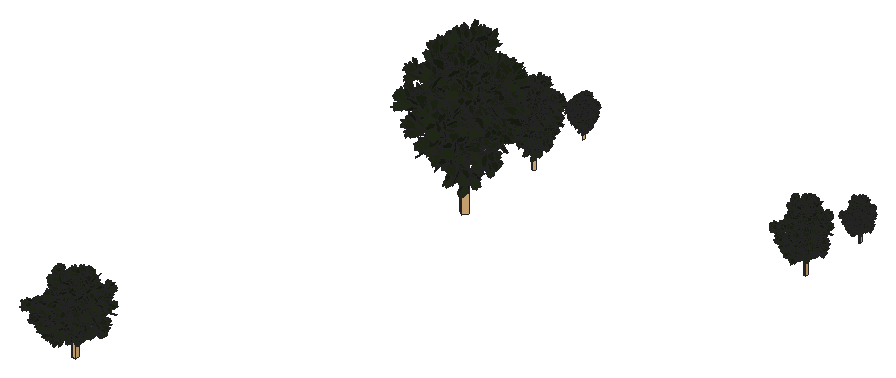
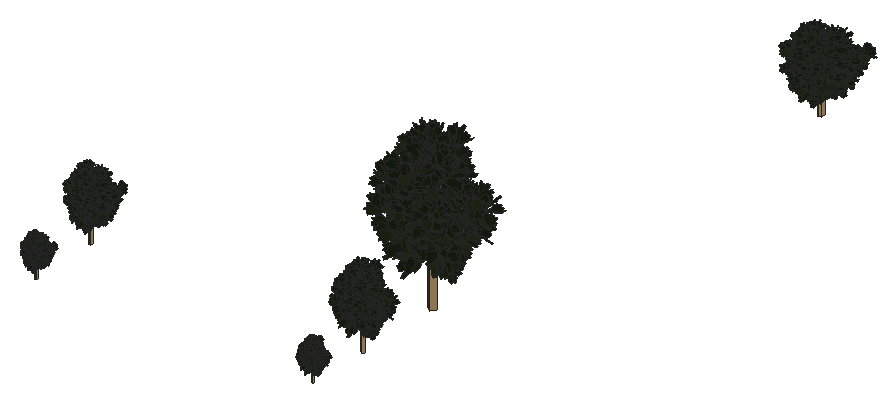
# SketchUp Ruby script. Lengths in inches.
U = 1.inch
M = Sketchup.active_model
def pt(a) = Geom::Point3d.new(a.map { |v| v * U })
def face(e, loops, mat)
  f = e.add_face(loops[0].map { |a| pt(a) })
  loops[1..].each { |l| e.add_face(l.map { |a| pt(a) }).erase! }
  f.material = f.back_material = mat if mat
  f
end
# faces: each face lists its corners as indices into pts; further lists are holes
def faces(e, pts, list, mat = nil) = list.each { |f| face(e, (f[0].is_a?(Array) ? f : [f]).map { |l| l.map { |i| pts[i] } }, mat) }
# xy, xz, yz: faces in a plane at the given z, y or x. An outline is a flat list of corners, or four numbers for a rectangle; further outlines are holes
def ring(l) = l.size == 4 ? [[l[0], l[1]], [l[2], l[1]], [l[2], l[3]], [l[0], l[3]]] : l.each_slice(2).to_a
def flat(e, list, mat, &to3) = list.each { |f| face(e, (f[0].is_a?(Array) ? f : [f]).map { |l| ring(l).map { |u, v| to3.(u, v) } }, mat) }
def xy(e, z, list, mat = nil) = flat(e, list, mat) { |x, y| [x, y, z] }
def xz(e, y, list, mat = nil) = flat(e, list, mat) { |x, z| [x, y, z] }
def yz(e, x, list, mat = nil) = flat(e, list, mat) { |y, z| [x, y, z] }
def lines(e, pts, list) = list.each { |a, b| e.add_line(pt(pts[a]), pt(pts[b])) }
# prism: a flat outline (further loops are holes) pulled along v
def prism(e, loops, v, mat = nil)
  f = face(e, loops, mat); d = Geom::Vector3d.new(v.map { |x| x * U })
  f.pushpull(f.normal.samedirection?(d) ? d.length : -d.length)
end
def box(e, o, s, mat = nil) = prism(e, [[o, [o[0] + s[0], o[1], o[2]], [o[0] + s[0], o[1] + s[1], o[2]], [o[0], o[1] + s[1], o[2]]]], [0, 0, s[2]], mat)
def at(x, y, z, deg = 0) = Geom::Transformation.translation(pt([x, y, z])) * Geom::Transformation.rotation(ORIGIN, Z_AXIS, deg.degrees)
def axes(o, x, y, z) = Geom::Transformation.new([*x, 0, *y, 0, *z, 0, *pt(o).to_a, 1])
def part(name) = M.definitions.add(name)
# library, detail: a bought-in or finely detailed component or shape, given as its bounding box
def library(name, o, s) = part(name).tap { |d| box(d.entities, o, s) }
def detail(e, o, s) = box(e.add_group.entities, o, s)
def put(e, d, t, mat = nil) = e.add_instance(d, t).tap { |i| i.material = mat if mat }
def group(e, t, mat = nil) = e.add_group.tap { |g| g.transformation = t; g.material = mat if mat }.entities
root = M.entities
M.materials.add("Color_D09").color = [86, 59, 49]
M.materials.add("Green ash – green texture").color = [33, 41, 22]
M.materials.add("[Color_005]1").color = [114, 114, 114]
c1 = part("Component\#32")
xz(c1.entities,0,[[2.54,0,9.87,0.64,10.99,2.07,11.4,3.42,15.13,2.28,14.48,4.31,16.14,5.21,16.14,6.08,19.81,7.28,19.6,9.67,17.45,11.49,17.45,12.16,18.82,14.37,17.48,14.37,14.41,13.66,14.41,15.23,12.5625,17.49,9.84,15.21,8.9,13.85,7.74,13.625,7.35,12.68,6.87,13.02,6.35,12.27,5.92,10.47,4.2,7.42,2.84,6.89,0,2.38,0.07,1.59,2.8125,4.94,3.37,3.59,2.54,3.37,2.12,2.22]],"Green ash – green texture")
c2 = part("Component\#31")
xz(c2.entities,0,[[1.1,0,1.61,0,2.73,1.11,4.34,2.72,5.21,6.36,5.85,7.16,6.35,6.9375,6.85,8.05,8.03,8.05,8.625,9.25,10.11,11.7,9.56,13.83,9.56,15.84,7.83,15.84,6.03,14.37,5.31,16.54,4.4375,17.39,1.45,14.31,0,9.15,1.4,5.18,3.01,6.08,1.98,1.39]],"Green ash – green texture")
c3 = part("Component\#30")
put(c3.entities,c1,axes([0,7.77,0],[1,0,0],[0,0.89571,0.44464],[0,-0.44464,0.89571]))
put(c3.entities,c2,axes([2.15,6.37,5.26],[0.57629,-0.80824,0.12095],[0.79263,0.51673,-0.3236],[0.19905,0.28236,0.93843]))
c4 = part("Component\#33")
put(c4.entities,c3,axes([-4.97,-3.22,4.05],[0.69883,-0.69034,0.18725],[0.53248,0.3273,-0.7806],[0.47759,0.64522,0.59632]))
c5 = part("Component\#35")
put(c5.entities,c4,axes([0,5.2,2.2],[1,0,0],[0,0.90259,0.43051],[0,-0.43051,0.90259]))
c6 = part("leaf group 2")
put(c6.entities,c5,axes([-11.99,4.41,-4.35],[2.22014,-0.82385,1.14017],[1.36501,1.77637,-1.37441],[-0.33979,1.75315,1.92841]))
c7 = part("Component\#37")
put(c7.entities,c6,axes([-5.27,11.65,1.68],[-0.48323,0.10636,-0.43072],[-0.11515,-0.64511,-0.03012],[-0.42845,0.05342,0.49388]))
c8 = part("Component\#36")
xz(c8.entities,0,[[0.64,0,0,0.1875,4.21,2.81,8.59,4.11,12.8,4.11,19.57,2.81,12.8,3.73,8.59,3.73,4.21,2.3125]],"Color_D09")
c9 = part("Leaf cluster")
put(c9.entities,c7,axes([23.53,12.57,24.85],[0.06536,-0.90475,-0.42089],[0.61791,-0.2945,0.72901],[-0.78353,-0.30772,0.53981]))
put(c9.entities,c7,axes([22.7,12.25,24.83],[-0.47146,-0.89493,0.11311],[0.80135,-0.48549,-0.35888],[0.36776,-0.0521,0.90651]))
put(c9.entities,c7,axes([24.25,0.65,20.83],[0.8253,-0.50372,0.24924],[0.23848,0.71461,0.65749],[-0.51157,-0.48438,0.71194]))
put(c9.entities,c7,axes([23.54,-2.45,18.63],[0.04689,-0.92492,0.3511],[0.72122,-0.28285,-0.64421],[0.71641,0.2674,0.65188]))
put(c9.entities,c7,axes([22.39,16.15,27.04],[-0.5311,-0.82173,0.2419],[0.41574,0.01583,0.89559],[-0.77461,0.50499,0.40813]))
put(c9.entities,c8,axes([22.76,-5.09,13.48],[0,1.66539,0.44624],[-1.72414,0,0],[0,-0.44624,1.66539]))
c10 = part("Bare twig")
p = [[0,0,0.13],[0.41,0.77,0],[4.07,2.79,10.125],[3.73,2.15,10.23],[7.66,4.77,23.875],[7.4,4.27,23.96],
  [8.6875,5.26,35.99],[8.5,4.91,36.05],[8.32,4.9375,46.95],[8.21,4.74,46.98]]
faces(c10.entities,p,[[0,1,2,3],[3,2,4,5],[4,6,7,5],[6,8,9,7]],"[Color_005]1")
c11 = part("Leafy twig")
put(c11.entities,c10,axes([3.13,0.17,-0.45],[3.38032,6.88592,0.52481],[-5.85488,3.97559,0.303],[0,-1.35912,3.54524]))
put(c11.entities,c7,axes([0.37,31.375,148.94],[0.47772,0.64064,-1.51139],[2.85768,-0.62659,0.20284],[-0.43926,-3.3797,-0.3241]))
c12 = part("Leafy branch")
put(c12.entities,c9,axes([28.11,72.66,46.26],[0.77413,-0.41274,-0.47998],[0.6311,0.56229,0.53435],[0.04934,-0.71657,0.69577]))
put(c12.entities,c9,axes([31.25,3.94,9.17],[0.73236,0.67893,0.05208],[-0.46223,0.55185,-0.69413],[-0.5,0.48428,0.71797]))
put(c12.entities,c9,axes([20.16,84.84,57.95],[0.96628,0.19619,0.16678],[-0.2575,0.73909,0.62245],[-0.00115,-0.6444,0.76469]))
put(c12.entities,c9,axes([30.13,29.18,11.93],[0.86603,0.2796,0.41452],[0,0.82904,-0.55919],[-0.5,0.48428,0.71797]))
put(c12.entities,c9,axes([47.67,28.63,-3.7],[0.1205,-0.71255,0.69119],[0.96646,0.24327,0.08231],[-0.2268,0.65809,0.71797]))
put(c12.entities,c9,axes([48.76,50.64,76.31],[-0.6716,0.46861,-0.57389],[0.01402,0.78248,0.62252],[0.74078,0.41004,-0.53209]))
put(c12.entities,c11,axes([42.34,0,10.34],[0.39368,0,0],[0,0.22544,-0.24092],[0,0.54032,0.50562]))
put(c12.entities,c9,axes([64.51,80.82,101.08],[-0.99604,0.06562,-0.06004],[-0.0106,0.58266,0.81265],[0.08831,0.81006,-0.57966]))
c13 = part("Leafy branch \#2")
put(c13.entities,c9,axes([-3.64,36.17,23.18],[0.95801,0.10249,0.26779],[-0.28581,0.41631,0.86313],[-0.02302,-0.90343,0.42812]))
put(c13.entities,c9,axes([13.16,55.79,39.92],[0.70711,-0.61725,0.34497],[0,0.48786,0.87292],[-0.70711,-0.61725,0.34497]))
put(c13.entities,c11,axes([18.8125,5.17,0.46],[0.25503,0,0],[0,0.20007,-0.0752],[0,0.16866,0.44872]))
put(c13.entities,c9,axes([23.62,-10.17,21.5],[-0.56253,0.81775,0.12181],[0.38738,0.13053,0.91263],[0.73041,0.56057,-0.39021]))
put(c13.entities,c9,axes([45.18,27.18,68.96],[-0.96593,-0.22593,0.12627],[0.12295,0.02876,0.992],[-0.22775,0.97372,0]))
c14 = library("Tree trunk",[-6.35,9.4375,-76.57],[12.56,13.68,315.77])
c15 = part("Leafy branch \#3")
put(c15.entities,c11,axes([21.47,3.93,0.22],[0.25503,0,0],[0,0.21068,-0.03601],[0,0.08077,0.47252]))
put(c15.entities,c9,axes([-4.05,13.6875,55.34],[0.70711,0.70373,-0.069],[0,0.09758,0.99523],[0.70711,-0.70373,0.069]))
put(c15.entities,c9,axes([6.52,33.54,18.07],[0.92587,-0.37604,0.03687],[0,0.09758,0.99523],[-0.37784,-0.92145,0.09035]))
c16 = part("Leafy branch \#1")
put(c16.entities,c9,axes([26.17,74.02,40.56],[0.25882,-0.64004,0.72344],[0,0.74896,0.66262],[-0.96593,-0.1715,0.19384]))
put(c16.entities,c9,axes([6.38,24.03,55.81],[-0.04786,0.8645,-0.50035],[0.15558,0.50126,0.85119],[0.98666,-0.03711,-0.15849]))
put(c16.entities,c11,axes([17.68,0,1.01],[0.32282,0,0],[0,0.21407,-0.16545],[0,0.37107,0.48011]))
put(c16.entities,c9,axes([-9.1875,31.15,28.07],[0.82314,0.37626,-0.42529],[0,0.74896,0.66262],[0.56784,-0.54543,0.61649]))
put(c16.entities,c9,axes([0.54,-12.07,9.94],[0.19622,0.90478,-0.37799],[-0.67396,0.40444,0.61823],[0.71224,0.13344,0.68914]))
put(c16.entities,c9,axes([7.34,9.15,39.57],[0.05153,0.73872,-0.67204],[0.38679,0.60565,0.6954],[0.92072,-0.29578,-0.25452]))
put(c16.entities,c9,axes([36.2,51.23,15.73],[-0.18626,-0.35374,0.91661],[-0.31641,0.90483,0.2849],[-0.93016,-0.23696,-0.28046]))
c17 = part("Tree")
put(c17.entities,c12,axes([209.16,146.26,190.79],[-0.28773,1.46382,-0.87256],[-1.6259,0,0.48096],[0.49836,0.84514,1.51132]))
put(c17.entities,c12,axes([134.38,215.25,141.01],[1.59145,0,0],[0,1.58386,0.23671],[0,-0.32836,1.69393]))
put(c17.entities,c13,axes([178.04,237.71,388.46],[0,-1.63474,0],[1.63474,0,0],[0,0,1.78187]))
put(c17.entities,c12,axes([256.65,171.18,211.31],[-1.36815,1.04036,0],[-1.04036,-1.36815,0],[0,0,1.87346]))
put(c17.entities,c12,axes([167.11,160.33,284.63],[0.63716,1.20925,-0.47341],[-1.25908,0.71729,0.13762],[0.43501,0.34501,1.46674]))
put(c17.entities,c14,axes([199.97,188.06,127.43],[1.59145,0,0],[0,1.59145,0],[0,0,1.66425]))
put(c17.entities,c12,axes([275.77,218.4,281.93],[-1.57517,-0.28132,-0.44593],[0.06295,-1.50318,0.62621],[-0.42383,0.67416,1.53786]))
put(c17.entities,c12,axes([190.14,288,146.64],[0.35111,-1.78964,0],[1.72866,0.33915,0.47202],[-0.50488,-0.09905,1.92016]))
put(c17.entities,c12,axes([257.54,236.65,165.53],[-1.29152,-0.54158,0],[0.54158,-1.29152,0],[0,0,1.52652]))
put(c17.entities,c12,axes([175.36,274.13,265.04],[0.47642,-1.31213,-0.12271],[1.30597,0.45529,0.24003],[-0.16973,-0.17989,1.50253]))
put(c17.entities,c13,axes([228.65,212.14,385.35],[-1.53723,0.39369,-0.12111],[-0.39786,-1.55122,0.00748],[-0.10661,0.11241,1.71849]))
put(c17.entities,c15,axes([179.375,247.82,455.73],[0.79573,-1.37824,0],[1.37824,0.79573,0],[0,0,1.73468]))
put(c17.entities,c15,axes([220.2,190.4,436.52],[-0.90108,1.29724,0.19482],[-1.26794,-0.9219,0.27414],[0.36658,0,1.69551]))
put(c17.entities,c16,axes([195.4,185.625,330.61],[0,1.80471,0],[-1.731,0,0.5105],[0.55644,0,1.88679]))
put(c17.entities,c16,axes([180.07,237.23,322.66],[1.03006,-1.73903,-0.39964],[1.71651,0.8636,0.79163],[-0.4607,-0.67055,2.05597]))
put(c17.entities,c12,axes([252.86,167.09,121.2],[-1.29065,1.04142,0.30989],[-1.03312,-1.28343,0.15838],[0.47872,-0.11505,1.68865]))
put(c17.entities,c12,axes([145.45,238.15,252.03],[1.32497,-0.45364,0],[0.45364,1.32497,0],[0,0,1.52652]))
put(c17.entities,c16,axes([222.54,228.83,294],[-1.20488,-1.04179,0.83261],[1.23186,-1.24114,0.27288],[0.38905,0.70343,1.7146]))
put(c17.entities,c16,axes([223.77,224.36,314.875],[-1.40575,-0.68986,-0.30962],[0.56266,-1.37824,0.6133],[-0.4899,0.39658,1.59284]))
put(c17.entities,c16,axes([166.75,216.1,346.53],[1.65511,0,0],[0,1.6365,0.2475],[0,-0.26977,1.78379]))
put(c17.entities,c13,axes([162.33,209.39,372.71],[1.56679,-0.27909,0],[0.27909,1.56679,0],[0,0,1.73468]))
put(c17.entities,c13,axes([203.35,171.86,386.35],[0.15996,1.63137,0],[-1.63137,0.15996,0],[0,0,1.78672]))
c18 = part("Green Ash")
put(c18.entities,c14,axes([99.99,94.03,63.71],[0.79573,0,0],[0,0.79573,0],[0,0,0.83213]))
put(c18.entities,c13,axes([101.67,85.93,193.17],[0.07998,0.81569,0],[-0.81569,0.07998,0],[0,0,0.89336]))
put(c18.entities,c13,axes([89.02,118.86,194.23],[0,-0.81737,0],[0.81737,0,0],[0,0,0.89093]))
put(c18.entities,c12,axes([137.88,109.2,140.96],[-0.78759,-0.14066,-0.22296],[0.03147,-0.75159,0.31311],[-0.21191,0.33708,0.76893]))
put(c18.entities,c12,axes([67.1875,107.625,70.5],[0.79573,0,0],[0,0.79193,0.11835],[0,-0.16418,0.84696]))
put(c18.entities,c12,axes([104.58,73.13,95.39],[-0.14386,0.73191,-0.43628],[-0.81295,0,0.24048],[0.24918,0.42257,0.75566]))
put(c18.entities,c12,axes([128.33,85.59,105.66],[-0.68407,0.52018,0],[-0.52018,-0.68407,0],[0,0,0.93673]))
put(c18.entities,c12,axes([128.77,118.32,82.77],[-0.64576,-0.27079,0],[0.27079,-0.64576,0],[0,0,0.76326]))
put(c18.entities,c13,axes([114.32,106.07,192.67],[-0.76861,0.19684,-0.06056],[-0.19893,-0.77561,0.00374],[-0.0533,0.05621,0.85925]))
put(c18.entities,c12,axes([83.56,80.16,142.32],[0.31858,0.60462,-0.23671],[-0.62954,0.35865,0.06881],[0.21751,0.1725,0.73337]))
put(c18.entities,c13,axes([81.16,104.7,186.36],[0.7834,-0.13954,0],[0.13954,0.7834,0],[0,0,0.86734]))
put(c18.entities,c16,axes([97.7,92.8125,165.31],[0,0.90235,0],[-0.8655,0,0.25525],[0.27822,0,0.94339]))
put(c18.entities,c12,axes([87.68,137.07,132.52],[0.23821,-0.65607,-0.06135],[0.65299,0.22764,0.12002],[-0.08486,-0.08995,0.75126]))
put(c18.entities,c15,axes([89.6875,123.91,227.86],[0.39786,-0.68912,0],[0.68912,0.39786,0],[0,0,0.86734]))
put(c18.entities,c12,axes([95.07,144,73.32],[0.17556,-0.89482,0],[0.86433,0.16957,0.23601],[-0.25244,-0.04953,0.96008]))
put(c18.entities,c15,axes([110.1,95.2,218.26],[-0.45054,0.64862,0.09741],[-0.63397,-0.46095,0.13707],[0.18329,0,0.84775]))
put(c18.entities,c16,axes([90.03,118.62,161.33],[0.51503,-0.86951,-0.19982],[0.85825,0.4318,0.39581],[-0.23035,-0.33528,1.02798]))
put(c18.entities,c16,axes([83.38,108.05,173.27],[0.82756,0,0],[0,0.81825,0.12375],[0,-0.13489,0.89189]))
put(c18.entities,c16,axes([111.27,114.42,147],[-0.60244,-0.5209,0.41631],[0.61593,-0.62057,0.13644],[0.19452,0.35171,0.8573]))
put(c18.entities,c12,axes([126.43,83.55,60.6],[-0.64533,0.52071,0.15494],[-0.51656,-0.64172,0.07919],[0.23936,-0.05752,0.84432]))
put(c18.entities,c16,axes([111.89,112.18,157.4375],[-0.70287,-0.34493,-0.15481],[0.28133,-0.68912,0.30665],[-0.24495,0.19829,0.79642]))
put(c18.entities,c12,axes([72.73,119.08,126.01],[0.66249,-0.22682,0],[0.22682,0.66249,0],[0,0,0.76326]))
put(root,c17,axes([382.22,636.45,-58.64],[0.2591,0.38413,0],[-0.38413,0.2591,0],[0,0,0.46335]))
put(root,c17,axes([365.36,857.42,-58.64],[0.12955,0.19207,0],[-0.19207,0.12955,0],[0,0,0.23167]))
put(root,c18,axes([789.44,879.81,-56.86],[0.4026,0,0],[0,0.4026,0],[0,0,0.4026]))
put(root,c18,axes([169,0,-20.14],[0.61,0,0],[0,0.61,0],[0,0,0.4514]))
put(root,c18,axes([805.9,1018.55,-58.6875],[0.23351,0,0],[0,0.23351,0],[0,0,0.23351]))
put(root,c17,axes([358.37,999.43,-58.64],[0.06477,0.09603,0],[-0.09603,0.06477,0],[0,0,0.11584]))
